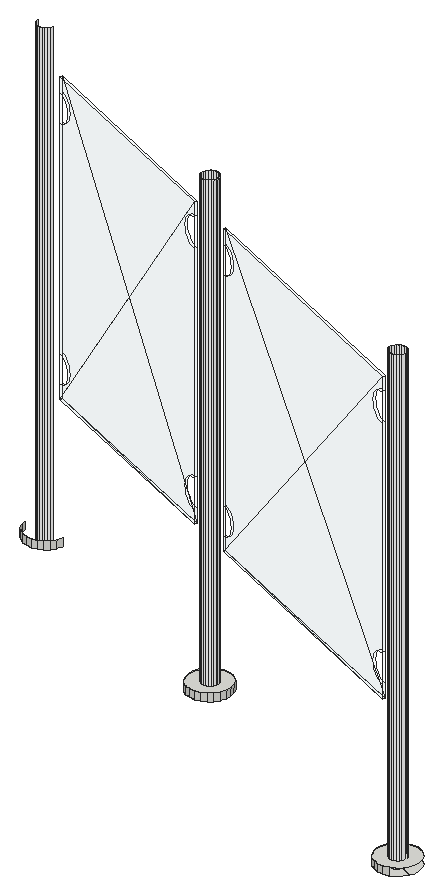
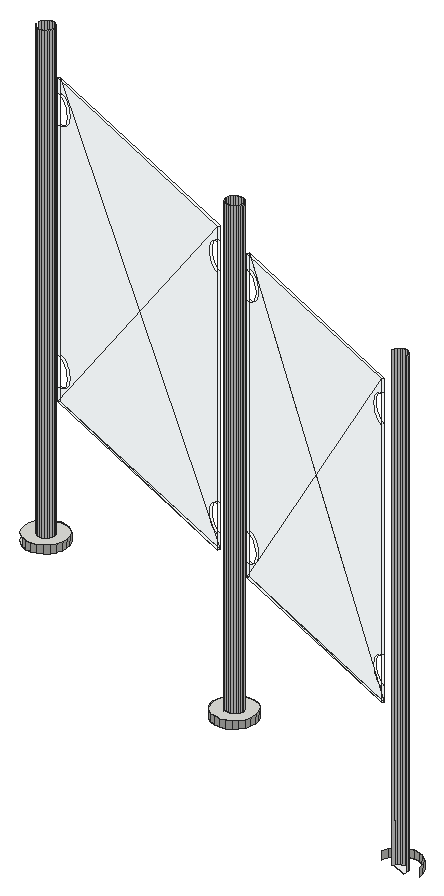
# SketchUp Ruby script. Lengths in inches.
U = 1.inch
M = Sketchup.active_model
def pt(a) = Geom::Point3d.new(a.map { |v| v * U })
def face(e, loops, mat)
  f = e.add_face(loops[0].map { |a| pt(a) })
  loops[1..].each { |l| e.add_face(l.map { |a| pt(a) }).erase! }
  f.material = f.back_material = mat if mat
  f
end
# faces: each face lists its corners as indices into pts; further lists are holes
def faces(e, pts, list, mat = nil) = list.each { |f| face(e, (f[0].is_a?(Array) ? f : [f]).map { |l| l.map { |i| pts[i] } }, mat) }
# xy, xz, yz: faces in a plane at the given z, y or x. An outline is a flat list of corners, or four numbers for a rectangle; further outlines are holes
def ring(l) = l.size == 4 ? [[l[0], l[1]], [l[2], l[1]], [l[2], l[3]], [l[0], l[3]]] : l.each_slice(2).to_a
def flat(e, list, mat, &to3) = list.each { |f| face(e, (f[0].is_a?(Array) ? f : [f]).map { |l| ring(l).map { |u, v| to3.(u, v) } }, mat) }
def xy(e, z, list, mat = nil) = flat(e, list, mat) { |x, y| [x, y, z] }
def xz(e, y, list, mat = nil) = flat(e, list, mat) { |x, z| [x, y, z] }
def yz(e, x, list, mat = nil) = flat(e, list, mat) { |y, z| [x, y, z] }
def lines(e, pts, list) = list.each { |a, b| e.add_line(pt(pts[a]), pt(pts[b])) }
# prism: a flat outline (further loops are holes) pulled along v
def prism(e, loops, v, mat = nil)
  f = face(e, loops, mat); d = Geom::Vector3d.new(v.map { |x| x * U })
  f.pushpull(f.normal.samedirection?(d) ? d.length : -d.length)
end
def box(e, o, s, mat = nil) = prism(e, [[o, [o[0] + s[0], o[1], o[2]], [o[0] + s[0], o[1] + s[1], o[2]], [o[0], o[1] + s[1], o[2]]]], [0, 0, s[2]], mat)
def at(x, y, z, deg = 0) = Geom::Transformation.translation(pt([x, y, z])) * Geom::Transformation.rotation(ORIGIN, Z_AXIS, deg.degrees)
def axes(o, x, y, z) = Geom::Transformation.new([*x, 0, *y, 0, *z, 0, *pt(o).to_a, 1])
def part(name) = M.definitions.add(name)
# library, detail: a bought-in or finely detailed component or shape, given as its bounding box
def library(name, o, s) = part(name).tap { |d| box(d.entities, o, s) }
def detail(e, o, s) = box(e.add_group.entities, o, s)
def put(e, d, t, mat = nil) = e.add_instance(d, t).tap { |i| i.material = mat if mat }
def group(e, t, mat = nil) = e.add_group.tap { |g| g.transformation = t; g.material = mat if mat }.entities
root = M.entities
M.materials.add("Glass_Safety_01").color = [204, 235, 244]
M.materials["Glass_Safety_01"].alpha = 0.1
M.materials.add("[Color_000]").color = [255, 255, 255]
xy(root,321.27,[[[674.38,606.04,674.79,606.125,675.15,606.31,675.46,606.58,675.6875,606.92,675.71,606.99,675.82,607.3125,675.84,607.72,675.76,608.13,675.58,608.49,675.3,608.8,674.96,609.03,674.57,609.16,674.16,609.18,673.76,609.1,673.39,608.92,673.08,608.64,672.86,608.3,672.83,608.24,672.73,607.91,672.7,607.5,672.78,607.1,672.97,606.73,673.24,606.42,673.58,606.2,673.97,606.07],[674.32,606.98,674.15,606.99,674,607.05,673.86,607.14,673.75,607.26,673.68,607.41,673.64,607.57,673.65,607.73,673.7,607.86,673.71,607.89,673.8,608.02,673.92,608.13,674.07,608.21,674.23,608.24,674.39,608.23,674.55,608.18,674.68,608.09,674.79,607.96,674.87,607.82,674.9,607.66,674.89,607.49,674.85,607.36,674.84,607.34,674.75,607.2,674.625,607.09,674.48,607.02]],[675.71,606.99,675.82,607.3125,675.84,607.72,675.76,608.13,675.58,608.49,675.3,608.8,674.96,609.03,674.57,609.16,674.16,609.18,673.76,609.1,673.39,608.92,673.08,608.64,672.86,608.3,672.83,608.24,673.7,607.86,673.71,607.89,673.8,608.02,673.92,608.13,674.07,608.21,674.23,608.24,674.39,608.23,674.55,608.18,674.68,608.09,674.79,607.96,674.87,607.82,674.9,607.66,674.89,607.49,674.85,607.36],[674.85,607.36,674.89,607.49,674.9,607.66,674.87,607.82,674.79,607.96,674.68,608.09,674.55,608.18,674.39,608.23,674.23,608.24,674.07,608.21,673.92,608.13,673.8,608.02,673.71,607.89,673.7,607.86],[[651.81,615.87,652.22,615.95,652.59,616.14,652.89,616.41,653.12,616.75,653.14,616.82,653.25,617.14,653.27,617.55,653.19,617.96,653.01,618.32,652.73,618.63,652.39,618.86,652,618.99,651.59,619.01,651.1875,618.93,650.82,618.75,650.51,618.47,650.29,618.13,650.16,617.74,650.13,617.33,650.21,616.93,650.4,616.56,650.67,616.25,651.01,616.02,651.4,615.9],[651.75,616.8125,651.58,616.82,651.43,616.875,651.29,616.97,651.18,617.09,651.11,617.24,651.07,617.4,651.08,617.5625,651.13,617.69,651.14,617.72,651.23,617.85,651.35,617.96,651.5,618.04,651.66,618.07,651.82,618.06,651.98,618.01,652.11,617.92,652.22,617.79,652.3,617.65,652.33,617.49,652.32,617.32,652.28,617.19,652.27,617.17,652.18,617.03,652.06,616.92,651.91,616.85]],[653.14,616.82,653.25,617.14,653.27,617.55,653.19,617.96,653.01,618.32,652.73,618.63,652.39,618.86,652,618.99,651.59,619.01,651.1875,618.93,650.82,618.75,650.51,618.47,650.29,618.13,650.27,618.07,651.13,617.69,651.14,617.72,651.23,617.85,651.35,617.96,651.5,618.04,651.66,618.07,651.82,618.06,651.98,618.01,652.11,617.92,652.22,617.79,652.3,617.65,652.33,617.49,652.32,617.32,652.28,617.19],
  [652.28,617.19,652.32,617.32,652.33,617.49,652.3,617.65,652.22,617.79,652.11,617.92,651.98,618.01,651.82,618.06,651.66,618.07,651.5,618.04,651.35,617.96,651.23,617.85,651.14,617.72,651.13,617.69]])
xy(root,321.27,[[674.32,606.98,674.48,607.02,674.625,607.09,674.75,607.2,674.84,607.34,674.85,607.36,673.7,607.86,673.65,607.73,673.64,607.57,673.68,607.41,673.75,607.26,673.86,607.14,674,607.05,674.15,606.99],[651.75,616.8125,651.91,616.85,652.06,616.92,652.18,617.03,652.27,617.17,652.28,617.19,651.13,617.69,651.08,617.5625,651.07,617.4,651.11,617.24,651.18,617.09,651.29,616.97,651.43,616.875,651.58,616.82],[632.1,625.37,632.26,625.4,632.41,625.48,632.53,625.59,632.625,625.72,632.63,625.75,631.48,626.25,631.4375,626.12,631.43,625.95,631.46,625.79,631.54,625.64,631.64,625.52,631.78,625.43,631.9375,625.38]],"[Color_000]")
xy(root,321.86,[[674.38,606.04,674.79,606.125,675.15,606.31,675.46,606.58,675.6875,606.92,675.82,607.3125,675.84,607.72,675.76,608.13,675.58,608.49,675.3,608.8,674.96,609.03,674.57,609.16,674.16,609.18,673.76,609.1,673.39,608.92,673.08,608.64,672.86,608.3,672.73,607.91,672.7,607.5,672.78,607.1,672.97,606.73,673.24,606.42,673.58,606.2,673.97,606.07],[651.81,615.87,652.22,615.95,652.59,616.14,652.89,616.41,653.12,616.75,653.25,617.14,653.27,617.55,653.19,617.96,653.01,618.32,652.73,618.63,652.39,618.86,652,618.99,651.59,619.01,651.1875,618.93,650.82,618.75,650.51,618.47,650.29,618.13,650.16,617.74,650.13,617.33,650.21,616.93,650.4,616.56,650.67,616.25,651.01,616.02,651.4,615.9]])
xy(root,331.9,[[672.57,608.24,653.47,616.57,653.55,616.75],[672.57,608.24,653.55,616.75,672.65,608.43],[650.02,618.07,633.82,625.12,633.9,625.3],[650.02,618.07,633.9,625.3,650.1,618.25]],"Glass_Safety_01")
p = [[673.97,606.07,321.27],[674.38,606.04,321.27],[674.38,606.04,321.86],[673.97,606.07,321.86],[674.79,606.125,321.27],[674.79,606.125,321.86],
  [673.58,606.2,321.27],[673.58,606.2,321.86],[673.24,606.42,321.27],[673.24,606.42,321.86],[672.97,606.73,321.27],[672.97,606.73,321.86],
  [672.78,607.1,321.27],[672.78,607.1,321.86],[673.86,607.14,321.27],[674,607.05,321.27],[674,607.05,357.27],[673.86,607.14,357.27],
  [674.15,606.99,321.27],[674.15,606.99,357.27],[674.32,606.98,321.27],[674.32,606.98,357.27],[674.48,607.02,321.27],[674.48,607.02,357.27],
  [674.625,607.09,321.27],[674.625,607.09,357.27],[672.7,607.5,321.27],[672.7,607.5,321.86],[673.75,607.26,321.27],[673.75,607.26,357.27],
  [674.75,607.2,321.27],[674.75,607.2,357.27],[674.84,607.34,321.27],[674.84,607.34,357.27],[673.68,607.41,321.27],[673.68,607.41,357.27],
  [674.85,607.36,321.27],[674.89,607.49,321.27],[674.89,607.49,357.27],[673.64,607.57,321.27],[673.64,607.57,357.27],[672.73,607.91,321.27],
  [672.73,607.91,321.86],[673.65,607.73,321.27],[673.65,607.73,357.27],[673.71,607.89,321.27],[673.7,607.86,321.27],[673.71,607.89,357.27],
  [674.87,607.82,321.27],[674.79,607.96,321.27],[674.79,607.96,357.27],[674.87,607.82,357.27],[672.86,608.3,321.27],[672.83,608.24,321.27],
  [672.86,608.3,321.86],[673.8,608.02,321.27],[673.8,608.02,357.27],[673.92,608.13,321.27],[673.92,608.13,357.27],[674.68,608.09,321.27],
  [674.68,608.09,357.27],[674.07,608.21,321.27],[674.07,608.21,357.27],[674.55,608.18,321.27],[674.55,608.18,357.27],[674.23,608.24,321.27],
  [674.23,608.24,357.27],[674.39,608.23,321.27],[674.39,608.23,357.27],[673.08,608.64,321.27],[673.08,608.64,321.86],[673.39,608.92,321.27],
  [673.39,608.92,321.86],[673.76,609.1,321.27],[673.76,609.1,321.86],[674.96,609.03,321.27],[674.57,609.16,321.27],[674.57,609.16,321.86],
  [674.96,609.03,321.86],[674.16,609.18,321.27],[674.16,609.18,321.86],[651.01,616.02,321.27],[651.4,615.9,321.27],[651.4,615.9,321.86],
  [651.01,616.02,321.86],[651.81,615.87,321.27],[651.81,615.87,321.86],[652.22,615.95,321.27],[652.22,615.95,321.86],[650.67,616.25,321.27],
  [650.67,616.25,321.86],[652.59,616.14,321.27],[652.59,616.14,321.86],[652.89,616.41,321.27],[652.89,616.41,321.86],[650.4,616.56,321.27],
  [650.4,616.56,321.86],[653.12,616.75,321.27],[653.12,616.75,321.86],[650.21,616.93,321.27],[650.21,616.93,321.86],[651.43,616.875,321.27],
  [651.58,616.82,321.27],[651.58,616.82,357.27],[651.43,616.875,357.27],[651.75,616.8125,321.27],[651.75,616.8125,357.27],[651.91,616.85,321.27],
  [651.91,616.85,357.27],[652.06,616.92,321.27],[652.06,616.92,357.27],[653.14,616.82,321.27],[653.25,617.14,321.27],[653.25,617.14,321.86],
  [650.13,617.33,321.27],[650.13,617.33,321.86],[651.29,616.97,321.27],[651.29,616.97,357.27],[652.18,617.03,321.27],[652.18,617.03,357.27],
  [651.18,617.09,321.27],[651.18,617.09,357.27],[652.27,617.17,321.27],[652.27,617.17,357.27],[651.11,617.24,321.27],[651.11,617.24,357.27],
  [653.27,617.55,321.27],[653.27,617.55,321.86],[651.07,617.4,321.27],[651.07,617.4,357.27],[652.28,617.19,321.27],[652.32,617.32,321.27],
  [652.32,617.32,357.27],[650.16,617.74,321.27],[650.16,617.74,321.86],[652.33,617.49,321.27],[652.33,617.49,357.27],[651.08,617.5625,321.27],
  [651.08,617.5625,357.27],[652.3,617.65,321.27],[652.3,617.65,357.27],[651.14,617.72,321.27],[651.13,617.69,321.27],[651.14,617.72,357.27],
  [652.22,617.79,321.27],[652.22,617.79,357.27],[653.19,617.96,321.27],[653.19,617.96,321.86],[650.29,618.13,321.27],[650.27,618.07,321.27],
  [650.29,618.13,321.86],[651.23,617.85,321.27],[651.23,617.85,357.27],[652.11,617.92,321.27],[652.11,617.92,357.27],[651.35,617.96,321.27],
  [651.35,617.96,357.27],[651.98,618.01,321.27],[651.98,618.01,357.27],[651.5,618.04,321.27],[651.5,618.04,357.27],[651.66,618.07,321.27],
  [651.66,618.07,357.27],[651.82,618.06,321.27],[651.82,618.06,357.27],[653.01,618.32,321.27],[653.01,618.32,321.86],[650.51,618.47,321.27],
  [650.51,618.47,321.86],[652.73,618.63,321.27],[652.73,618.63,321.86],[650.82,618.75,321.27],[650.82,618.75,321.86],[652.39,618.86,321.27],
  [652.39,618.86,321.86],[651.1875,618.93,321.27],[651.1875,618.93,321.86],[651.59,619.01,321.27],[651.59,619.01,321.86],[652,618.99,321.27],
  [652,618.99,321.86],[631.76,624.45,321.27],[632.17,624.43,321.27],[632.17,624.43,321.86],[631.76,624.45,321.86],[632.57,624.51,321.27],
  [632.57,624.51,321.86],[631.37,624.58,321.27],[631.37,624.58,321.86],[632.94,624.69,321.27],[632.94,624.69,321.86],[631.03,624.81,321.27],
  [631.03,624.81,321.86],[633.25,624.97,321.27],[633.25,624.97,321.86],[630.75,625.11,321.27],[630.75,625.11,321.86],[633.47,625.31,321.27],
  [633.47,625.31,321.86],[630.57,625.48,321.27],[630.57,625.48,321.86],[633.49,625.37,321.27],[633.6,625.7,321.27],[633.6,625.7,321.86],
  [631.64,625.52,321.27],[631.78,625.43,321.27],[631.78,625.43,357.27],[631.64,625.52,357.27],[631.9375,625.38,321.27],[631.9375,625.38,357.27],
  [632.1,625.37,321.27],[632.1,625.37,357.27],[632.26,625.4,321.27],[632.26,625.4,357.27],[632.41,625.48,321.27],[632.41,625.48,357.27],
  [630.49,625.89,321.27],[630.49,625.89,321.86],[631.54,625.64,321.27],[631.54,625.64,357.27],[632.53,625.59,321.27],[632.53,625.59,357.27],
  [631.46,625.79,321.27],[631.46,625.79,357.27],[632.625,625.72,321.27],[632.625,625.72,357.27],[632.63,625.75,321.27],[632.68,625.88,321.27],
  [632.68,625.88,357.27],[631.43,625.95,321.27],[631.43,625.95,357.27],[653.47,616.57,351.28],[653.47,616.57,335.125],[653.72,616.46,335.09],
  [653.96,616.35,334.98],[654.16,616.27,334.8125],[654.3125,616.2,334.59],[654.41,616.16,334.34],[654.44,616.14,334.0625],[654.41,616.16,333.79],
  [654.3125,616.2,333.53],[654.16,616.27,333.3125],[653.96,616.35,333.14],[653.72,616.46,333.04],[653.47,616.57,333],[653.47,616.57,331.9],
  [672.57,608.24,354.51],[653.47,616.57,354.51],[653.47,616.57,353.41],[653.72,616.46,353.37],[653.96,616.35,353.27],[654.16,616.27,353.1],
  [654.3125,616.2,352.88],[654.41,616.16,352.62],[654.44,616.14,352.35],[654.41,616.16,352.07],[654.3125,616.2,351.81],[654.16,616.27,351.59],
  [653.96,616.35,351.43],[653.72,616.46,351.32],[672.57,608.24,331.9],[672.57,608.24,333],[672.43,608.31,333],[672.18,608.42,333.04],
  [671.94,608.52,333.14],[671.74,608.61,333.3125],[671.58,608.68,333.53],[671.49,608.72,333.79],[671.45,608.73,334.0625],[671.49,608.72,334.34],
  [671.58,608.68,334.59],[671.74,608.61,334.8125],[671.94,608.52,334.98],[672.18,608.42,335.09],[672.43,608.31,335.125],[672.57,608.24,335.125],
  [672.57,608.24,351.28],[672.43,608.31,351.28],[672.18,608.42,351.32],[671.94,608.52,351.43],[671.74,608.61,351.59],[671.58,608.68,351.81],
  [671.49,608.72,352.07],[671.45,608.73,352.35],[671.49,608.72,352.62],[671.58,608.68,352.88],[671.74,608.61,353.1],[671.94,608.52,353.27],
  [672.18,608.42,353.37],[672.43,608.31,353.41],[672.57,608.24,353.41],[672.65,608.43,331.9],[672.65,608.43,333],[672.65,608.43,335.125],
  [672.65,608.43,351.28],[672.65,608.43,353.41],[672.65,608.43,354.51],[653.55,616.75,331.9],[653.55,616.75,333],[653.8,616.64,333.04],
  [654.03,616.53,333.14],[654.24,616.45,333.3125],[654.39,616.38,333.53],[654.49,616.34,333.79],[654.52,616.32,334.0625],[654.49,616.34,334.34],
  [654.39,616.38,334.59],[654.24,616.45,334.8125],[654.03,616.53,334.98],[653.8,616.64,335.09],[653.55,616.75,335.125],[653.55,616.75,351.28],
  [653.8,616.64,351.32],[654.03,616.53,351.43],[654.24,616.45,351.59],[654.39,616.38,351.81],[654.49,616.34,352.07],[654.52,616.32,352.35],
  [654.49,616.34,352.62],[654.39,616.38,352.88],[654.24,616.45,353.1],[654.03,616.53,353.27],[653.8,616.64,353.37],[653.55,616.75,353.41],
  [653.55,616.75,354.51],[672.51,608.49,335.125],[672.25,608.6,335.09],[672.02,608.7,334.98],[671.82,608.79,334.8125],[671.66,608.86,334.59],
  [671.57,608.9,334.34],[671.53,608.91,334.0625],[671.57,608.9,333.79],[671.66,608.86,333.53],[671.82,608.79,333.3125],[672.02,608.7,333.14],
  [672.25,608.6,333.04],[672.51,608.49,333],[672.51,608.49,353.41],[672.25,608.6,353.37],[672.02,608.7,353.27],[671.82,608.79,353.1],
  [671.66,608.86,352.88],[671.57,608.9,352.62],[671.53,608.91,352.35],[671.57,608.9,352.07],[671.66,608.86,351.81],[671.82,608.79,351.59],
  [672.02,608.7,351.43],[672.25,608.6,351.32],[672.51,608.49,351.28],[633.82,625.12,351.28],[633.82,625.12,335.125],[634.07,625.01,335.09],
  [634.31,624.91,334.98],[634.51,624.82,334.8125],[634.67,624.75,334.59],[634.76,624.71,334.34],[634.8,624.7,334.0625],[634.76,624.71,333.79],
  [634.67,624.75,333.53],[634.51,624.82,333.3125],[634.31,624.91,333.14],[634.07,625.01,333.04],[633.82,625.12,333],[633.82,625.12,331.9],
  [650.02,618.07,354.51],[633.82,625.12,354.51],[633.82,625.12,353.41],[634.07,625.01,353.37],[634.31,624.91,353.27],[634.51,624.82,353.1],
  [634.67,624.75,352.88],[634.76,624.71,352.62],[634.8,624.7,352.35],[634.76,624.71,352.07],[634.67,624.75,351.81],[634.51,624.82,351.59],
  [634.31,624.91,351.43],[634.07,625.01,351.32],[650.02,618.07,331.9],[650.02,618.07,333],[649.86,618.14,333],[649.61,618.25,333.04],
  [649.37,618.35,333.14],[649.17,618.4375,333.3125],[649.01,618.5,333.53],[648.92,618.55,333.79],[648.88,618.5625,334.0625],[648.92,618.55,334.34],
  [649.01,618.5,334.59],[649.17,618.4375,334.8125],[649.37,618.35,334.98],[649.61,618.25,335.09],[649.86,618.14,335.125],[650.02,618.07,335.125],
  [650.02,618.07,351.28],[649.86,618.14,351.28],[649.61,618.25,351.32],[649.37,618.35,351.43],[649.17,618.4375,351.59],[649.01,618.5,351.81],
  [648.92,618.55,352.07],[648.88,618.5625,352.35],[648.92,618.55,352.62],[649.01,618.5,352.88],[649.17,618.4375,353.1],[649.37,618.35,353.27],
  [649.61,618.25,353.37],[649.86,618.14,353.41],[650.02,618.07,353.41],[650.1,618.25,331.9],[650.1,618.25,333],[650.1,618.25,335.125],
  [650.1,618.25,351.28],[650.1,618.25,353.41],[650.1,618.25,354.51],[633.9,625.3,331.9],[633.9,625.3,333],[634.15,625.19,333.04],
  [634.39,625.09,333.14],[634.59,625,333.3125],[634.75,624.93,333.53],[634.84,624.89,333.79],[634.875,624.88,334.0625],[634.84,624.89,334.34],
  [634.75,624.93,334.59],[634.59,625,334.8125],[634.39,625.09,334.98],[634.15,625.19,335.09],[633.9,625.3,335.125],[633.9,625.3,351.28],
  [634.15,625.19,351.32],[634.39,625.09,351.43],[634.59,625,351.59],[634.75,624.93,351.81],[634.84,624.89,352.07],[634.875,624.88,352.35],
  [634.84,624.89,352.62],[634.75,624.93,352.88],[634.59,625,353.1],[634.39,625.09,353.27],[634.15,625.19,353.37],[633.9,625.3,353.41],
  [633.9,625.3,354.51],[649.9375,618.32,335.125],[649.68,618.43,335.09],[649.45,618.53,334.98],[649.25,618.62,334.8125],[649.09,618.69,334.59],
  [649,618.73,334.34],[648.96,618.74,334.0625],[649,618.73,333.79],[649.09,618.69,333.53],[649.25,618.62,333.3125],[649.45,618.53,333.14],
  [649.68,618.43,333.04],[649.9375,618.32,333],[649.9375,618.32,353.41],[649.68,618.43,353.37],[649.45,618.53,353.27],[649.25,618.62,353.1],
  [649.09,618.69,352.88],[649,618.73,352.62],[648.96,618.74,352.35],[649,618.73,352.07],[649.09,618.69,351.81],[649.25,618.62,351.59],
  [649.45,618.53,351.43],[649.68,618.43,351.32],[649.9375,618.32,351.28]]
faces(root,p,[[0,1,2,3],[1,4,5,2],[6,0,3,7],[8,6,7,9],[10,8,9,11],[12,10,11,13],[26,12,13,27],[41,26,27,42],
  [52,53,41,42,54],[69,52,54,70],[71,69,70,72],[73,71,72,74],[75,76,77,78],[79,73,74,80],[76,79,80,77],[81,82,83,84],
  [82,85,86,83],[85,87,88,86],[89,81,84,90],[87,91,92,88],[91,93,94,92],[95,89,90,96],[93,97,98,94],[99,95,96,100],
  [97,111,112,113,98],[114,99,100,115],[112,126,127,113],[133,114,115,134],[126,146,147,127],[148,149,133,134,150],[146,165,166,147],[167,148,150,168],
  [165,169,170,166],[171,167,168,172],[169,173,174,170],[175,171,172,176],[177,175,176,178],[173,179,180,174],[179,177,178,180],[181,182,183,184],
  [182,185,186,183],[187,181,184,188],[185,189,190,186],[191,187,188,192],[189,193,194,190],[195,191,192,196],[193,197,198,194],[199,195,196,200],
  [197,201,202,203,198],[216,199,200,217]])
faces(root,p,[[14,15,16,17],[15,18,19,16],[18,20,21,19],[20,22,23,21],[22,24,25,23],[28,14,17,29],[24,30,31,25],[30,32,33,31],
  [34,28,29,35],[32,36,37,38,33],[39,34,35,40],[43,39,40,44],[45,46,43,44,47],[48,49,50,51],[55,45,47,56],[57,55,56,58],
  [49,59,60,50],[61,57,58,62],[59,63,64,60],[65,61,62,66],[67,65,66,68],[63,67,68,64],[101,102,103,104],[102,105,106,103],
  [105,107,108,106],[107,109,110,108],[116,101,104,117],[109,118,119,110],[120,116,117,121],[118,122,123,119],[124,120,121,125],[128,124,125,129],
  [122,130,131,132,123],[131,135,136,132],[137,128,129,138],[135,139,140,136],[141,142,137,138,143],[139,144,145,140],[151,141,143,152],[144,153,154,145],
  [155,151,152,156],[153,157,158,154],[159,155,156,160],[161,159,160,162],[157,163,164,158],[163,161,162,164],[204,205,206,207],[205,208,209,206],
  [208,210,211,209],[210,212,213,211],[212,214,215,213],[218,204,207,219],[214,220,221,215],[222,218,219,223],[220,224,225,221],[224,226,227,228,225],
  [229,222,223,230]],"[Color_000]")
faces(root,p,[[231,232,233,234,235,236,237,238,239,240,241,242,243,244,245,246,247,248,249,250,251,252,253,254,255,256,257,258,259],[260,261,262,263,264,265,266,267,268,269,270,271,272,273,274,275,276,277,278,279,280,281,282,283,284,285,286,287,288,289,290,246,245],[260,291,292,293,294,295,296,246,290,276,275,261],[297,298,299,300,301,302,303,304,305,306,307,308,309,310,311,312,313,314,315,316,317,318,319,320,321,322,323,324,291],[294,293,325,326,327,328,329,330,331,332,333,334,335,336,337,292,291,324,296,295,338,339,340,341,342,343,344,345,346,347,348,349,350],[297,245,244,232,231,248,247,324,323,311,310,298],[351,352,353,354,355,356,357,358,359,360,361,362,363,364,365,366,367,368,369,370,371,372,373,374,375,376,377,378,379],[380,381,382,383,384,385,386,387,388,389,390,391,392,393,394,395,396,397,398,399,400,401,402,403,404,405,406,407,408,409,410,366,365],
  [380,411,412,413,414,415,416,366,410,396,395,381],[417,418,419,420,421,422,423,424,425,426,427,428,429,430,431,432,433,434,435,436,437,438,439,440,441,442,443,444,411],[414,413,445,446,447,448,449,450,451,452,453,454,455,456,457,412,411,444,416,415,458,459,460,461,462,463,464,465,466,467,468,469,470],[417,365,364,352,351,368,367,444,443,431,430,418]],"Glass_Safety_01")
